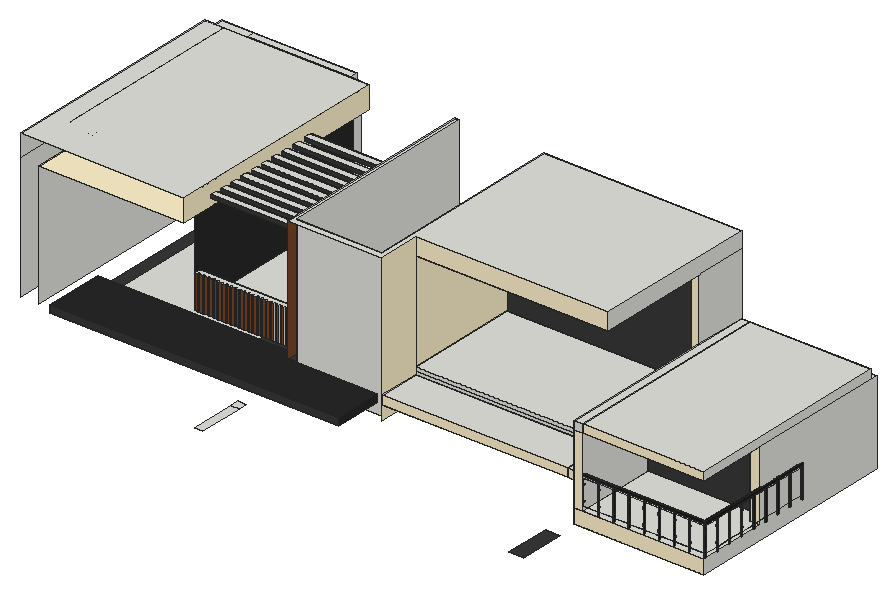
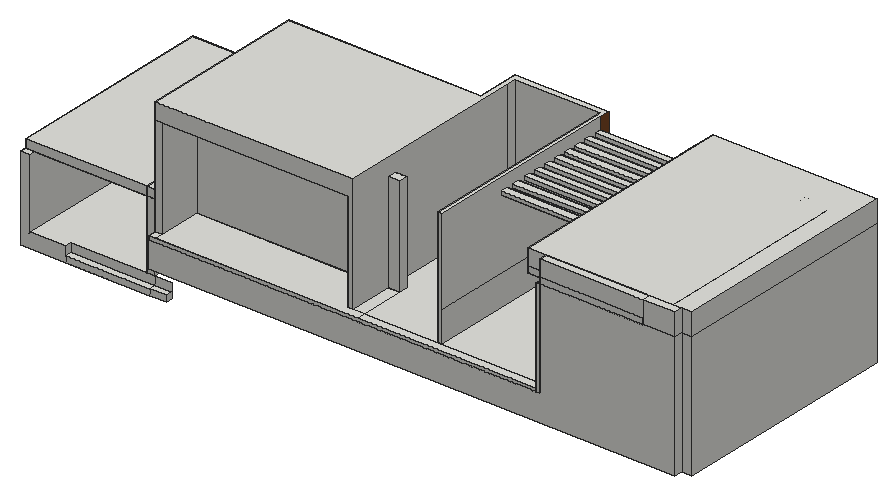
# SketchUp Ruby script. Lengths in inches.
U = 1.inch
M = Sketchup.active_model
def pt(a) = Geom::Point3d.new(a.map { |v| v * U })
def face(e, loops, mat)
  f = e.add_face(loops[0].map { |a| pt(a) })
  loops[1..].each { |l| e.add_face(l.map { |a| pt(a) }).erase! }
  f.material = f.back_material = mat if mat
  f
end
# faces: each face lists its corners as indices into pts; further lists are holes
def faces(e, pts, list, mat = nil) = list.each { |f| face(e, (f[0].is_a?(Array) ? f : [f]).map { |l| l.map { |i| pts[i] } }, mat) }
# xy, xz, yz: faces in a plane at the given z, y or x. An outline is a flat list of corners, or four numbers for a rectangle; further outlines are holes
def ring(l) = l.size == 4 ? [[l[0], l[1]], [l[2], l[1]], [l[2], l[3]], [l[0], l[3]]] : l.each_slice(2).to_a
def flat(e, list, mat, &to3) = list.each { |f| face(e, (f[0].is_a?(Array) ? f : [f]).map { |l| ring(l).map { |u, v| to3.(u, v) } }, mat) }
def xy(e, z, list, mat = nil) = flat(e, list, mat) { |x, y| [x, y, z] }
def xz(e, y, list, mat = nil) = flat(e, list, mat) { |x, z| [x, y, z] }
def yz(e, x, list, mat = nil) = flat(e, list, mat) { |y, z| [x, y, z] }
def lines(e, pts, list) = list.each { |a, b| e.add_line(pt(pts[a]), pt(pts[b])) }
# prism: a flat outline (further loops are holes) pulled along v
def prism(e, loops, v, mat = nil)
  f = face(e, loops, mat); d = Geom::Vector3d.new(v.map { |x| x * U })
  f.pushpull(f.normal.samedirection?(d) ? d.length : -d.length)
end
def box(e, o, s, mat = nil) = prism(e, [[o, [o[0] + s[0], o[1], o[2]], [o[0] + s[0], o[1] + s[1], o[2]], [o[0], o[1] + s[1], o[2]]]], [0, 0, s[2]], mat)
def at(x, y, z, deg = 0) = Geom::Transformation.translation(pt([x, y, z])) * Geom::Transformation.rotation(ORIGIN, Z_AXIS, deg.degrees)
def axes(o, x, y, z) = Geom::Transformation.new([*x, 0, *y, 0, *z, 0, *pt(o).to_a, 1])
def part(name) = M.definitions.add(name)
# library, detail: a bought-in or finely detailed component or shape, given as its bounding box
def library(name, o, s) = part(name).tap { |d| box(d.entities, o, s) }
def detail(e, o, s) = box(e.add_group.entities, o, s)
def put(e, d, t, mat = nil) = e.add_instance(d, t).tap { |i| i.material = mat if mat }
def group(e, t, mat = nil) = e.add_group.tap { |g| g.transformation = t; g.material = mat if mat }.entities
root = M.entities
M.materials.add("[0131_Silver]").color = [28, 28, 28]
M.materials.add("[Color D01]").color = [255, 242, 204]
M.materials.add("[Color M08]").color = [56, 56, 56]
M.materials.add("[Granite Dark Gray]").color = [40, 40, 40]
M.materials.add("[Translucent_Glass_Blue]").color = [255, 255, 255]
M.materials["[Translucent_Glass_Blue]"].alpha = 0
M.materials.add("[Wood Floor Dark]").color = [153, 94, 42]
M.materials.add("[Wood Veneer 01]").color = [120, 70, 37]
c1 = part("Group\#11")
xy(c1.entities,0,[[0,0,0.39,2.125]],"[0131_Silver]")
xy(c1.entities,1.5,[[0,0,0.39,2.125]],"[0131_Silver]")
xz(c1.entities,0,[[0,0,0.39,1.5]],"[0131_Silver]")
xz(c1.entities,2.125,[[0,0,0.39,1.5]],"[0131_Silver]")
yz(c1.entities,0,[[0,0,2.125,1.5]],"[0131_Silver]")
yz(c1.entities,0.39,[[0,0,2.125,1.5]],"[0131_Silver]")
c2 = part("Glass railing panel")
xy(c2.entities,0,[[-0.59,0,0,63.98]])
xy(c2.entities,37.71,[[-0.59,0,0,63.98]])
xz(c2.entities,0,[[-0.59,0,0,37.71]])
xz(c2.entities,63.98,[[-0.59,0,0,37.71]])
yz(c2.entities,-0.59,[[0,0,63.98,37.71]])
yz(c2.entities,0,[[0,0,63.98,0,63.98,37.71,0,37.71,0,30.53,1.75,30.53,1.75,28.71,0,28.71],[-0.4,28.71,0,30.53],[0,28.71,1.75,30.53]])
p = [[0,63.98,30.53],[0.39,63.98,30.53]]
lines(c2.entities,p,[[0,1]])
put(c2.entities,c1,axes([0,62.22,28.71],[1,0,0],[0,1.01246,0],[0,0,1.2158]))
put(c2.entities,c1,axes([0,62.22,6.27],[1,0,0],[0,1.01246,0],[0,0,1.2158]))
put(c2.entities,c1,axes([0,0.6,28.71],[1,0,0],[0,1.01246,0],[0,0,1.2158]))
put(c2.entities,c1,axes([0,0.6,6.27],[1,0,0],[0,1.01246,0],[0,0,1.2158]))
put(c2.entities,c1,axes([-0.98,0.6,28.71],[1,0,0],[0,1.01246,0],[0,0,1.2158]))
put(c2.entities,c1,axes([-0.98,62.22,6.27],[1,0,0],[0,1.01246,0],[0,0,1.2158]))
put(c2.entities,c1,axes([-0.98,0.6,6.27],[1,0,0],[0,1.01246,0],[0,0,1.2158]))
put(c2.entities,c1,axes([-0.98,62.22,28.71],[1,0,0],[0,1.01246,0],[0,0,1.2158]))
c3 = part("Group\#1")
xz(c3.entities,0,[[0,0,1.97,38.58]])
xz(c3.entities,1.97,[[0,0,1.97,38.58]])
yz(c3.entities,0,[[0,0,1.97,37.71]])
yz(c3.entities,1.97,[[0,0,1.97,37.71]])
c4 = part("Glass railing")
xy(c4.entities,37.71,[[2.51,0,3.15,0.39,3.15,0]])
xy(c4.entities,37.71,[[0,0,0.54,520.67],[2.51,0,2.51,63.58,3.15,0.39],[3.15,0.39,2.51,63.58,2.51,520.67,3.15,520.67]],"[0131_Silver]")
xy(c4.entities,38.58,[[0.54,496.0625,2.51,520.67]])
xy(c4.entities,38.58,[[0.54,0,2.51,496.0625]],"[0131_Silver]")
xy(c4.entities,40.46,[[0,0,3.15,520.67]],"[0131_Silver]")
xz(c4.entities,0,[[0,37.71,0.54,37.71,0.54,38.58,2.51,38.58,2.51,37.71,3.15,37.71,3.15,40.46,0,40.46]],"[0131_Silver]")
xz(c4.entities,520.67,[[0,37.71,0,40.46,3.15,40.46,3.15,37.71,2.51,37.71,2.51,38.58,0.54,38.58,0.54,37.71]])
yz(c4.entities,0,[[0,37.71,520.67,40.46]],"[0131_Silver]")
yz(c4.entities,0.54,[[496.0625,37.71,520.67,38.58]])
yz(c4.entities,0.54,[[0,37.71,496.0625,38.58]],"[0131_Silver]")
yz(c4.entities,2.51,[[0,37.71,496.0625,38.58],[496.0625,37.71,520.67,38.58]])
yz(c4.entities,3.15,[[0,37.71,520.67,40.46]],"[0131_Silver]")
put(c4.entities,c2,axes([1.8,65.35,3.9375],[1,0,0],[0,0.98769,0],[0,0,0.8225]),"[Translucent_Glass_Blue]")
put(c4.entities,c2,axes([1.8,130.31,3.9375],[1,0,0],[0,0.98769,0],[0,0,0.8225]),"[Translucent_Glass_Blue]")
put(c4.entities,c2,axes([1.8,195.28,3.9375],[1,0,0],[0,0.98769,0],[0,0,0.8225]),"[Translucent_Glass_Blue]")
put(c4.entities,c2,axes([1.8,260.24,3.9375],[1,0,0],[0,0.98769,0],[0,0,0.8225]),"[Translucent_Glass_Blue]")
put(c4.entities,c2,axes([1.8,325.2,3.9375],[1,0,0],[0,0.98769,0],[0,0,0.8225]),"[Translucent_Glass_Blue]")
put(c4.entities,c2,axes([1.8,390.16,3.9375],[1,0,0],[0,0.98769,0],[0,0,0.8225]),"[Translucent_Glass_Blue]")
put(c4.entities,c2,axes([1.8,455.12,3.9375],[1,0,0],[0,0.98769,0],[0,0,0.8225]),"[Translucent_Glass_Blue]")
put(c4.entities,c2,axes([1.8,0.39,3.9375],[1,0,0],[0,0.98769,0],[0,0,0.8225]),"[Translucent_Glass_Blue]")
put(c4.entities,c3,at(0.54,128.9375,0),"[0131_Silver]")
g1 = group(c4.entities,at(0.54,63.98,0),"[0131_Silver]")
xz(g1,0,[[0,0,1.97,38.58]])
xz(g1,1.97,[[0,0,1.97,38.58]])
yz(g1,0,[[0,0,1.97,37.71]])
yz(g1,1.97,[[0,0,1.97,37.71]])
put(c4.entities,c3,at(0.54,193.9,0),"[0131_Silver]")
put(c4.entities,c3,at(0.54,258.86,0),"[0131_Silver]")
put(c4.entities,c3,at(0.54,323.82,0),"[0131_Silver]")
put(c4.entities,c3,at(0.54,388.78,0),"[0131_Silver]")
put(c4.entities,c3,at(0.54,453.74,0),"[0131_Silver]")
put(c4.entities,c3,at(0.54,518.7,0),"[0131_Silver]")
c5 = part("Glass+Railing (1)")
put(c5.entities,c4,axes([0,0,0],[1,0,0],[0,0.95652,0],[0,0,1]),"[0131_Silver]")
xy(root,291.625,[[1127.04,401,1272.34,411.84],[1272.34,401,1283.18,411.84],[1283.18,401,1286.86,411.84],[1286.86,401,1350.48,411.84],[1272.34,411.84,1283.18,687.48],
  [1283.18,411.84,1286.86,687.48],[1098.24,687.48,1272.34,698.3125],[1272.34,687.48,1283.18,698.3125],[1283.18,687.48,1286.86,698.3125],[1286.86,687.48,1350.48,698.3125]])
xy(root,291.625,[[1127.04,328.1875,1272.34,401],[1272.34,328.1875,1283.18,401],[1283.18,328.1875,1350.48,401],[1286.86,411.84,1350.48,687.48]],"[Color D01]")
xy(root,291.625,[[1107.49,212.24,1132.55,290.49]],"[Color M08]")
xy(root,293.375,[[566.56,212.24,581.07,290.49],[566.56,290.49,581.07,305]])
xy(root,302.375,[[1098.24,687.48,1127.04,698.3125],[1127.04,687.48,1272.34,698.3125]])
xy(root,316.5625,[[1127.04,328.1875,1141.52,687.48],[1141.52,328.1875,1350.48,328.1875,1350.48,446.91,1333.68,446.91,1333.68,468.95,1141.52,468.95],[1141.52,485.48,1333.68,485.48,1333.68,698.3125,1272.34,698.3125,1272.34,687.48,1141.52,687.48]])
xy(root,333.5625,[[787.31,411.84,787.31,687.48,1116.92,687.48,1116.92,411.84,1110.75,411.84,1110.75,652.46,796.43,652.46,796.43,411.84]])
xy(root,333.5625,[[796.43,401,796.43,652.46,1110.75,652.46,1110.75,411.84,1108.3,411.84,1108.3,401]],"[Color M08]")
xy(root,342.3125,[[307.88,347.0625,540.88,356.52]])
xy(root,342.3125,[[282.79,356.52,641.68,687.48]],"[Color M08]")
xy(root,345.5,[[307.88,356.52,540.88,566.77]])
xy(root,359.12,[[1115.11,328.1875,1126.93,401]])
xy(root,359.12,[[796.43,328.1875,1115.11,401]],"[Color D01]")
xy(root,359.31,[[291.49,245.0625,291.49,347.0625,634.74,347.0625,634.74,328.1875,787.93,328.1875,787.93,245.0625]],"[Granite Dark Gray]")
xy(root,372.12,[[291.49,245.0625,787.93,245.0625,787.93,328.1875,634.74,328.1875,634.74,347.0625,291.49,347.0625]],"[Granite Dark Gray]")
xy(root,373.17,[[796.43,328.1875,1115.11,401],[1115.11,328.1875,1126.93,401]])
xy(root,378.9375,[[460.02,345.0625,466.19,347.0625],[468.21,345.0625,474.38,347.0625],[476.52,345.0625,482.69,347.0625],[484.84,345.0625,491.01,347.0625],[492.96,345.0625,499.13,347.0625],
  [500.52,345.0625,506.69,347.0625],[508.09,345.0625,514.26,347.0625],[515.65,345.0625,521.82,347.0625],[523.21,345.0625,529.38,347.0625],[530.77,345.0625,536.94,347.0625],
  [538.34,345.0625,544.51,347.0625],[545.9,345.0625,552.07,347.0625],[553.46,345.0625,559.63,347.0625],[561.02,345.0625,567.19,347.0625],[568.59,345.0625,574.76,347.0625],
  [576.15,345.0625,582.32,347.0625],[583.71,345.0625,589.88,347.0625],[591.27,345.0625,597.44,347.0625],[599.77,345.0625,605.94,347.0625],[608.27,345.0625,614.44,347.0625],
  [616.77,345.0625,622.94,347.0625],[625.27,345.0625,631.44,347.0625],[460.02,347.0625,634.74,356.52],[460.02,356.52,634.74,401],[460.02,401,634.74,687.48],
  [634.74,401,796.43,687.48],[796.43,401,1127.04,401,1127.04,411.84,1116.92,411.84,1116.92,687.48,796.43,687.48],[1116.92,411.84,1127.04,687.48],[454.4,687.48,460.02,701.99],[460.02,687.48,1127.04,701.99]])
xy(root,385.6875,[[460.02,401,796.43,401,796.43,596.88,766.93,596.88,766.93,687.48,460.02,687.48],[796.43,401,1127.04,596.88],[766.93,596.88,796.43,612.82],[796.43,596.88,796.43,612.82,1114.68,612.82,1114.68,687.48,1127.04,687.48,1127.04,596.88],[766.93,612.82,1114.68,701.99],
  [460.02,687.48,766.93,701.99],[1114.68,687.48,1127.04,701.99]])
xy(root,436,[[1127.04,328.1875,1141.52,687.48],[1333.68,446.91,1333.68,468.95,1141.52,468.95,1141.52,485.48,1333.68,485.48,1333.68,687.48,1350.48,687.48,1350.48,446.91],[1141.52,485.48,1333.68,687.48],[1333.68,687.48,1350.48,698.3125]])
xy(root,436,[[1141.52,328.1875,1141.52,343.37,1335.3,343.37,1335.3,446.91,1350.48,446.91,1350.48,328.1875]],"[Color D01]")
xy(root,436,[[1141.52,343.37,1141.52,468.95,1333.68,468.95,1333.68,446.91,1335.3,446.91,1335.3,343.37]],"[Wood Floor Dark]")
xy(root,437.0625,[[460.02,345.0625,466.19,345.0625,466.19,347.0625,468.21,347.0625,468.21,345.0625,474.38,345.0625,474.38,347.0625,476.52,347.0625,476.52,345.0625,482.69,345.0625,482.69,347.0625,484.84,347.0625,484.84,345.0625,491.01,345.0625,491.01,347.0625,492.96,347.0625,492.96,345.0625,499.13,345.0625,499.13,347.0625,500.52,347.0625,500.52,345.0625,506.69,345.0625,506.69,347.0625,508.09,347.0625,508.09,345.0625,514.26,345.0625,514.26,347.0625,515.65,347.0625,515.65,345.0625,521.82,345.0625,521.82,347.0625,523.21,347.0625,523.21,345.0625,529.38,345.0625,529.38,347.0625,530.77,347.0625,530.77,345.0625,536.94,345.0625,536.94,347.0625,538.34,347.0625,538.34,345.0625,544.51,345.0625,544.51,347.0625,545.9,347.0625,545.9,345.0625,552.07,345.0625,552.07,347.0625,553.46,347.0625,553.46,345.0625,559.63,345.0625,559.63,347.0625,561.02,347.0625,561.02,345.0625,567.19,345.0625,567.19,347.0625,568.59,347.0625,568.59,345.0625,574.76,345.0625,574.76,347.0625,576.15,347.0625,576.15,345.0625,582.32,345.0625,582.32,347.0625,583.71,347.0625,583.71,345.0625,589.88,345.0625,589.88,347.0625,591.27,347.0625,591.27,345.0625,597.44,345.0625,597.44,347.0625,599.77,347.0625,599.77,345.0625,605.94,345.0625,605.94,347.0625,608.27,347.0625,608.27,345.0625,614.44,345.0625,614.44,347.0625,616.77,347.0625,616.77,345.0625,622.94,345.0625,622.94,347.0625,625.27,347.0625,625.27,345.0625,631.44,345.0625,631.44,347.0625,634.74,347.0625,634.74,356.52,460.02,356.52]])
xy(root,450.1875,[[1127.04,328.1875,1141.52,687.48],[1141.52,328.1875,1350.48,687.48]])
xy(root,546.625,[[236.62,290.49,485.87,687.48]],"[Color D01]")
xy(root,547.25,[[276.18,347.0625,276.18,701.99,454.4,701.99,454.4,687.48,282.79,687.48,282.79,347.0625],[282.79,347.0625,454.4,356.52],[454.4,347.0625,460.02,356.52],[460.02,347.0625,485.73,356.52],[282.79,356.52,454.4,687.48],
  [454.4,356.52,460.02,687.48],[460.02,356.52,485.73,687.48],[454.4,687.48,460.02,701.99]])
xy(root,556.88,[[766.93,596.88,796.43,612.82],[796.43,596.88,796.43,612.82,1114.68,612.82,1114.68,687.48,1127.04,687.48,1127.04,596.88],[796.43,612.82,1114.68,687.48]])
xy(root,556.88,[[796.43,401,1127.04,596.88]],"[Color D01]")
xy(root,559.64,[[485.87,498.22,634.74,510.59]],"[Color M08]")
xy(root,559.65,[[485.87,476.53,634.74,488.9]],"[Granite Dark Gray]")
xy(root,559.66,[[485.87,454.84,634.74,467.22]],"[Color M08]")
xy(root,559.66,[[485.87,433.15,634.74,445.53]],"[Granite Dark Gray]")
xy(root,559.67,[[485.87,411.47,634.74,423.84]],"[Granite Dark Gray]")
xy(root,559.68,[[485.87,389.78,634.74,402.15]],"[Color M08]")
xy(root,559.6875,[[485.87,368.09,634.74,380.47]],"[Color M08]")
xy(root,559.69,[[485.87,346.4,634.74,358.78],[485.87,523.15,634.74,535.53]],"[Granite Dark Gray]")
xy(root,559.74,[[485.87,548.09,634.74,560.47]],"[Color M08]")
xy(root,565.83,[[485.87,498.22,634.74,510.59]])
xy(root,565.84,[[485.87,454.84,634.74,467.22],[485.87,476.53,634.74,488.9]])
xy(root,565.85,[[485.87,433.15,634.74,445.53]])
xy(root,565.86,[[485.87,411.47,634.74,423.84]])
xy(root,565.87,[[485.87,389.78,634.74,402.15]])
xy(root,565.875,[[485.87,368.09,634.74,380.47]])
xy(root,565.88,[[485.87,346.4,634.74,358.78],[485.87,523.15,634.74,535.53]])
xy(root,565.93,[[485.87,548.09,634.74,560.47]])
xy(root,585.5,[[204.29,290.49,485.87,290.49,485.87,347.0625,485.73,347.0625,485.73,687.48,204.29,687.48],[634.74,328.1875,796.43,328.1875,796.43,401,1127.04,401,1127.04,687.48,787.31,687.48,787.31,338.65,641.68,338.65,641.68,687.48,634.74,687.48],[485.73,347.0625,485.87,356.52],[485.73,356.52,485.87,687.48],[222.11,687.48,276.18,701.99],
  [276.18,687.48,454.4,701.99]])
xz(root,245.0625,[[291.49,359.31,787.93,372.12]],"[Color M08]")
xz(root,328.1875,[[1127.04,436,1141.52,450.1875]])
xz(root,328.1875,[[1127.04,291.625,1350.48,316.5625],[1127.04,316.5625,1141.52,436],[796.43,359.12,1115.11,373.17],[1115.11,359.12,1126.93,373.17],[1141.52,436,1350.48,450.1875]],"[Color D01]")
xz(root,338.65,[[641.68,333.5625,787.31,585.5]])
xz(root,345.0625,[[460.02,378.9375,466.19,437.0625],[468.21,378.9375,474.38,437.0625],[476.52,378.9375,482.69,437.0625],[484.84,378.9375,491.01,437.0625],[492.96,378.9375,499.13,437.0625],
  [500.52,378.9375,506.69,437.0625],[508.09,378.9375,514.26,437.0625],[515.65,378.9375,521.82,437.0625],[523.21,378.9375,529.38,437.0625],[530.77,378.9375,536.94,437.0625],
  [538.34,378.9375,544.51,437.0625],[545.9,378.9375,552.07,437.0625],[553.46,378.9375,559.63,437.0625],[561.02,378.9375,567.19,437.0625],[568.59,378.9375,574.76,437.0625],
  [576.15,378.9375,582.32,437.0625],[583.71,378.9375,589.88,437.0625],[591.27,378.9375,597.44,437.0625],[599.77,378.9375,605.94,437.0625],[608.27,378.9375,614.44,437.0625],
  [616.77,378.9375,622.94,437.0625],[625.27,378.9375,631.44,437.0625]],"[Wood Veneer 01]")
xz(root,346.4,[[485.87,559.69,634.74,565.88]],"[Color M08]")
xz(root,347.0625,[[482.7,342.3125,482.86,359.31]],"[Granite Dark Gray]")
xz(root,347.0625,[[460.53,342.3125,463.64,359.31],[463.64,342.3125,464.34,359.31],[464.34,342.3125,467.45,359.31],[467.45,342.3125,468.15,359.31],[468.15,342.3125,471.27,359.31],
  [471.27,342.3125,471.97,359.31],[471.97,342.3125,475.08,359.31],[475.08,342.3125,475.78,359.31],[475.78,342.3125,478.89,359.31],[478.89,342.3125,479.59,359.31],
  [479.59,342.3125,482.7,359.31],[482.86,342.3125,485.86,359.31],[485.86,342.3125,486.67,359.31],[486.67,342.3125,489.68,359.31],[489.68,342.3125,490.49,359.31],
  [490.49,342.3125,493.49,359.31],[493.49,342.3125,494.3,359.31],[494.3,342.3125,497.3,359.31],[497.3,342.3125,498.11,359.31],[498.11,342.3125,501.11,359.31],
  [501.11,342.3125,501.92,359.31],[501.92,342.3125,504.93,359.31],[504.93,342.3125,505.74,359.31],[505.74,342.3125,508.74,359.31],[508.74,342.3125,509.55,359.31],
  [509.55,342.3125,512.55,359.31],[512.55,342.3125,513.36,359.31],[513.36,342.3125,516.36,359.31],[516.36,342.3125,517.17,359.31],[517.17,342.3125,520.18,359.31],
  [520.18,342.3125,520.99,359.31],[520.99,342.3125,523.99,359.31],[523.99,342.3125,524.8,359.31],[524.8,342.3125,527.8,359.31],[527.8,342.3125,528.61,359.31],
  [528.61,342.3125,531.61,359.31],[531.61,342.3125,532.67,359.31],[532.67,342.3125,535.68,359.31],[535.68,342.3125,536.49,359.31],[536.49,342.3125,539.49,359.31],
  [539.49,342.3125,540.88,359.31],[466.19,378.9375,468.21,437.0625],[474.38,378.9375,476.52,437.0625],[482.69,378.9375,484.84,437.0625],[491.01,378.9375,492.96,437.0625],
  [499.13,378.9375,500.52,437.0625],[506.69,378.9375,508.09,437.0625],[514.26,378.9375,515.65,437.0625],[521.82,378.9375,523.21,437.0625],[529.38,378.9375,530.77,437.0625],
  [536.94,378.9375,538.34,437.0625],[544.51,378.9375,545.9,437.0625],[552.07,378.9375,553.46,437.0625],[559.63,378.9375,561.02,437.0625],[567.19,378.9375,568.59,437.0625],
  [574.76,378.9375,576.15,437.0625],[582.32,378.9375,583.71,437.0625],[589.88,378.9375,591.27,437.0625],[597.44,378.9375,599.77,437.0625],[605.94,378.9375,608.27,437.0625],
  [614.44,378.9375,616.77,437.0625],[622.94,378.9375,625.27,437.0625],[631.44,378.9375,634.74,437.0625]],"[Wood Veneer 01]")
xz(root,356.52,[[307.88,342.3125,540.88,345.5],[460.02,378.9375,634.74,437.0625]])
xz(root,358.78,[[485.87,559.69,634.74,565.88]])
xz(root,368.09,[[485.87,559.6875,634.74,565.875]],"[Color M08]")
xz(root,380.47,[[485.87,559.6875,634.74,565.875]])
xz(root,389.78,[[485.87,559.68,634.74,565.87]],"[Color M08]")
xz(root,401,[[1115.11,291.625,1126.93,302.375],[1126.93,291.625,1127.04,302.375],[1115.11,302.375,1126.93,333.5625],[1126.93,302.375,1127.04,333.5625],[1126.93,333.5625,1127.04,333.5625,1127.04,378.9375,796.43,378.9375,796.43,373.17,1126.93,373.17],
  [1115.11,333.5625,1126.93,359.12],[796.43,359.12,1115.11,373.17],[1115.11,359.12,1126.93,373.17],[460.02,378.9375,796.43,385.6875],[796.43,378.9375,1127.04,385.6875]])
xz(root,401,[[796.43,556.88,1127.04,585.5]],"[Color D01]")
xz(root,401,[[796.43,333.5625,1115.11,359.12]],"[Granite Dark Gray]")
xz(root,402.15,[[485.87,559.68,634.74,565.87]])
xz(root,411.47,[[485.87,559.67,634.74,565.86]],"[Color M08]")
xz(root,411.84,[[1108.3,291.625,1110.75,316.5625],[1110.75,291.625,1116.92,316.5625],[1116.92,291.625,1127.04,316.5625],[1108.3,316.5625,1110.75,333.5625],[1110.75,316.5625,1116.92,333.5625],
  [1116.92,316.5625,1127.04,333.5625],[1116.92,333.5625,1127.04,378.9375]])
xz(root,423.84,[[485.87,559.67,634.74,565.86]])
xz(root,433.15,[[485.87,559.66,634.74,565.85]],"[Color M08]")
xz(root,445.53,[[485.87,559.66,634.74,565.85]])
xz(root,446.91,[[1333.68,316.5625,1350.48,436]],"[Color D01]")
xz(root,454.84,[[485.87,559.66,634.74,565.84]],"[Color M08]")
xz(root,467.22,[[485.87,559.66,634.74,565.84]])
xz(root,468.95,[[1141.52,316.5625,1333.68,436]],"[Color M08]")
xz(root,476.53,[[485.87,559.65,634.74,565.84]],"[Color M08]")
xz(root,485.48,[[1141.52,316.5625,1333.68,436]])
xz(root,488.9,[[485.87,559.65,634.74,565.84]])
xz(root,498.22,[[485.87,559.64,634.74,565.83]],"[Color M08]")
xz(root,510.59,[[485.87,559.64,634.74,565.83]])
xz(root,523.15,[[485.87,559.69,634.74,565.88]],"[Color M08]")
xz(root,535.53,[[485.87,559.69,634.74,565.88]])
xz(root,548.09,[[485.87,559.74,634.74,565.93]],"[Color M08]")
xz(root,560.47,[[485.87,559.74,634.74,565.93]])
xz(root,596.88,[[1114.68,385.6875,1127.04,556.88]],"[Color D01]")
xz(root,596.88,[[766.93,385.6875,1114.68,556.88]],"[Color M08]")
xz(root,612.82,[[766.93,385.6875,1114.68,556.88]])
xz(root,687.48,[[1098.24,302.375,1127.04,316.5625],[1127.04,302.375,1272.34,316.5625],[1127.04,316.5625,1141.52,436],[204.29,333.5625,222.11,547.25],[641.68,333.5625,787.31,378.9375],
  [787.31,333.5625,1116.92,378.9375],[1116.92,333.5625,1127.04,378.9375],[282.79,342.3125,641.68,342.3125,641.68,378.9375,454.4,378.9375,454.4,546.625,282.79,546.625],[454.4,378.9375,460.02,546.625],[634.74,378.9375,641.68,385.6875],
  [787.31,378.9375,787.31,585.5,1127.04,585.5,1127.04,556.88,796.43,556.88,796.43,378.9375],[634.74,385.6875,641.68,585.5],[1114.68,385.6875,1127.04,556.88],[1127.04,436,1141.52,450.1875],[1141.52,436,1350.48,450.1875],
  [282.79,546.625,454.4,547.25],[454.4,546.625,460.02,547.25],[460.02,546.625,460.02,547.25,485.73,547.25,485.73,585.5,485.87,585.5,485.87,546.625],[204.29,547.25,222.11,585.5],[282.79,547.25,454.4,557.875],
  [282.79,547.25,485.73,557.875],[454.4,547.25,485.73,557.875],[282.79,557.875,454.4,585.5],[454.4,557.875,485.73,585.5]])
xz(root,698.3125,[[1098.24,291.625,1127.04,302.375],[1127.04,291.625,1272.34,302.375],[1272.34,291.625,1272.34,316.5625,1333.68,316.5625,1333.68,436,1350.48,436,1350.48,291.625]])
xz(root,701.99,[[222.11,333.5625,222.11,547.25,454.4,547.25,454.4,378.9375,1127.04,378.9375,1127.04,333.5625],[454.4,378.9375,460.02,547.25],[460.02,378.9375,1127.04,385.6875],[222.11,547.25,276.18,585.5],[276.18,547.25,454.4,557.875],
  [276.18,557.875,454.4,585.5]])
yz(root,204.29,[[290.49,333.5625,687.48,547.25],[290.49,547.25,687.48,585.5]])
yz(root,222.11,[[687.48,333.5625,701.99,547.25],[687.48,547.25,701.99,585.5]])
yz(root,236.62,[[290.49,333.5625,687.48,546.625],[290.49,546.625,356.52,547.25]])
yz(root,276.18,[[347.0625,547.25,701.99,557.875]])
yz(root,282.79,[[347.0625,547.25,356.52,557.875],[356.52,547.25,687.48,557.875]])
yz(root,291.49,[[245.0625,359.31,347.0625,372.12]],"[Granite Dark Gray]")
yz(root,454.4,[[687.48,378.9375,701.99,547.25],[687.48,547.25,701.99,557.875],[687.48,557.875,701.99,585.5]])
yz(root,460.02,[[345.0625,378.9375,347.0625,437.0625],[347.0625,378.9375,356.52,437.0625],[401,378.9375,687.48,385.6875],[687.48,378.9375,701.99,385.6875],[687.48,385.6875,701.99,547.25]])
yz(root,460.02,[[356.52,378.9375,401,378.9375,401,385.6875,687.48,385.6875,687.48,547.25,347.0625,547.25,347.0625,437.0625,356.52,437.0625]],"[Granite Dark Gray]")
yz(root,466.19,[[345.0625,378.9375,347.0625,437.0625]])
yz(root,468.21,[[345.0625,378.9375,347.0625,437.0625]])
yz(root,474.38,[[345.0625,378.9375,347.0625,437.0625]])
yz(root,476.52,[[345.0625,378.9375,347.0625,437.0625]])
yz(root,482.69,[[345.0625,378.9375,347.0625,437.0625]])
yz(root,484.84,[[345.0625,378.9375,347.0625,437.0625]])
yz(root,485.73,[[347.0625,547.25,687.48,585.5]])
yz(root,485.87,[[[290.49,546.625,687.48,585.5],[346.4,559.69,358.78,565.88],[368.09,559.6875,380.47,565.875],[389.78,559.68,402.15,565.87],[411.47,559.67,423.84,565.86],[433.15,559.66,445.53,565.85],[454.84,559.66,467.22,565.84],[476.53,559.65,488.9,565.84],[498.22,559.64,510.59,565.83],[523.15,559.69,535.53,565.88],[548.09,559.74,560.47,565.93]]],"[Color D01]")
yz(root,491.01,[[345.0625,378.9375,347.0625,437.0625]])
yz(root,492.96,[[345.0625,378.9375,347.0625,437.0625]])
yz(root,499.13,[[345.0625,378.9375,347.0625,437.0625]])
yz(root,500.52,[[345.0625,378.9375,347.0625,437.0625]])
yz(root,506.69,[[345.0625,378.9375,347.0625,437.0625]])
yz(root,508.09,[[345.0625,378.9375,347.0625,437.0625]])
yz(root,514.26,[[345.0625,378.9375,347.0625,437.0625]])
yz(root,515.65,[[345.0625,378.9375,347.0625,437.0625]])
yz(root,521.82,[[345.0625,378.9375,347.0625,437.0625]])
yz(root,523.21,[[345.0625,378.9375,347.0625,437.0625]])
yz(root,529.38,[[345.0625,378.9375,347.0625,437.0625]])
yz(root,530.77,[[345.0625,378.9375,347.0625,437.0625]])
yz(root,536.94,[[345.0625,378.9375,347.0625,437.0625]])
yz(root,538.34,[[345.0625,378.9375,347.0625,437.0625]])
yz(root,544.51,[[345.0625,378.9375,347.0625,437.0625]])
yz(root,545.9,[[345.0625,378.9375,347.0625,437.0625]])
yz(root,552.07,[[345.0625,378.9375,347.0625,437.0625]])
yz(root,553.46,[[345.0625,378.9375,347.0625,437.0625]])
yz(root,559.63,[[345.0625,378.9375,347.0625,437.0625]])
yz(root,561.02,[[345.0625,378.9375,347.0625,437.0625]])
yz(root,567.19,[[345.0625,378.9375,347.0625,437.0625]])
yz(root,568.59,[[345.0625,378.9375,347.0625,437.0625]])
yz(root,574.76,[[345.0625,378.9375,347.0625,437.0625]])
yz(root,576.15,[[345.0625,378.9375,347.0625,437.0625]])
yz(root,582.32,[[345.0625,378.9375,347.0625,437.0625]])
yz(root,583.71,[[345.0625,378.9375,347.0625,437.0625]])
yz(root,589.88,[[345.0625,378.9375,347.0625,437.0625]])
yz(root,591.27,[[345.0625,378.9375,347.0625,437.0625]])
yz(root,597.44,[[345.0625,378.9375,347.0625,437.0625]])
yz(root,599.77,[[345.0625,378.9375,347.0625,437.0625]])
yz(root,605.94,[[345.0625,378.9375,347.0625,437.0625]])
yz(root,608.27,[[345.0625,378.9375,347.0625,437.0625]])
yz(root,614.44,[[345.0625,378.9375,347.0625,437.0625]])
yz(root,616.77,[[345.0625,378.9375,347.0625,437.0625]])
yz(root,622.94,[[345.0625,378.9375,347.0625,437.0625]])
yz(root,625.27,[[345.0625,378.9375,347.0625,437.0625]],"[Wood Veneer 01]")
yz(root,631.44,[[345.0625,378.9375,347.0625,437.0625]])
yz(root,634.74,[[347.0625,378.9375,356.52,437.0625],[356.52,378.9375,687.48,437.0625],[[347.0625,437.0625,347.0625,559.69,358.78,559.69,358.78,565.88,347.0625,565.88,347.0625,585.5,687.48,585.5,687.48,437.0625],[368.09,559.6875,380.47,565.875],[389.78,559.68,402.15,565.87],[411.47,559.67,423.84,565.86],[433.15,559.66,445.53,565.85],[454.84,559.66,467.22,565.84],[476.53,559.65,488.9,565.84],[498.22,559.64,510.59,565.83],[523.15,559.69,535.53,565.88],[548.09,559.74,560.47,565.93]],[346.4,559.69,347.0625,565.88],[347.0625,559.69,358.78,565.88]])
yz(root,634.74,[[328.1875,333.5625,347.0625,359.31]],"[Granite Dark Gray]")
yz(root,634.74,[[328.1875,372.12,328.1875,585.5,347.0625,585.5,347.0625,565.88,346.4,565.88,346.4,559.69,347.0625,559.69,347.0625,372.12]],"[Wood Veneer 01]")
yz(root,641.68,[[338.65,333.5625,356.52,333.5625,356.52,342.3125,687.48,342.3125,687.48,585.5,338.65,585.5]])
yz(root,766.93,[[596.88,385.6875,612.82,556.88]])
yz(root,787.31,[[338.65,333.5625,356.52,585.5],[356.52,333.5625,687.48,585.5]])
yz(root,787.93,[[245.0625,359.31,328.1875,372.12]],"[Granite Dark Gray]")
yz(root,796.43,[[328.1875,359.12,401,373.17],[401,378.9375,687.48,385.6875]])
yz(root,796.43,[[328.1875,333.5625,401,359.12],[328.1875,373.17,401,585.5],[401,385.6875,687.48,556.88]],"[Color D01]")
yz(root,1098.24,[[687.48,291.625,698.3125,302.375]])
yz(root,1114.68,[[612.82,385.6875,687.48,556.88]])
yz(root,1115.11,[[328.1875,359.12,401,373.17]])
yz(root,1116.92,[[411.84,333.5625,687.48,378.9375]])
yz(root,1126.93,[[328.1875,359.12,401,373.17]])
yz(root,1127.04,[[328.1875,291.625,401,316.5625],[401,291.625,411.84,316.5625],[328.1875,316.5625,401,436],[401,316.5625,411.84,378.9375],[411.84,316.5625,687.48,378.9375],
  [401,378.9375,411.84,385.6875],[411.84,378.9375,687.48,385.6875],[687.48,378.9375,701.99,385.6875],[401,385.6875,411.84,436],[411.84,385.6875,596.88,436],
  [596.88,385.6875,687.48,436],[328.1875,436,401,450.1875],[401,436,411.84,450.1875],[411.84,436,596.88,450.1875],[596.88,436,687.48,450.1875],
  [596.88,450.1875,687.48,556.88],[401,556.88,687.48,585.5]])
yz(root,1141.52,[[328.1875,316.5625,468.95,436],[468.95,316.5625,485.48,436],[485.48,316.5625,687.48,436],[328.1875,436,687.48,450.1875]])
yz(root,1272.34,[[687.48,302.375,698.3125,316.5625]])
yz(root,1333.68,[[446.91,316.5625,468.95,436],[485.48,316.5625,698.3125,436]])
yz(root,1350.48,[[328.1875,291.625,698.3125,291.625,698.3125,436,446.91,436,446.91,316.5625,328.1875,316.5625],[328.1875,436,687.48,450.1875]])
p = [[1333.68,701.95,316.5625],[1333.68,698.3125,316.5625],[1114.68,425.36,385.6875],[1114.68,596.88,385.6875],[787.31,687.48,385.6875],[766.93,687.48,385.6875],
  [276.18,347.0625,557.875],[276.18,347.0625,585.5],[282.79,347.0625,557.875],[282.79,347.0625,585.5],[282.79,356.52,557.875],[282.79,356.52,585.5],
  [236.62,356.52,547.25],[236.62,356.52,585.5],[460.02,356.52,546.625],[460.02,356.52,547.25],[485.87,356.52,547.25],[485.73,356.52,547.25],
  [236.62,356.52,546.625],[485.87,356.52,546.625],[236.62,687.48,585.5]]
lines(root,p,[[0,1],[2,3],[4,5],[6,7],[8,9],[10,11],[12,13],[14,15],[16,17],[14,18],[16,19],[13,20]])
put(root,c5,axes([1141.52,331.34,316.5625],[0,-1,0],[0.41958,0,0],[0,0,1.41]))
put(root,c5,axes([1350.48,328.1875,316.5625],[1,0,0],[0,0.41958,0],[0,0,1.41]))
